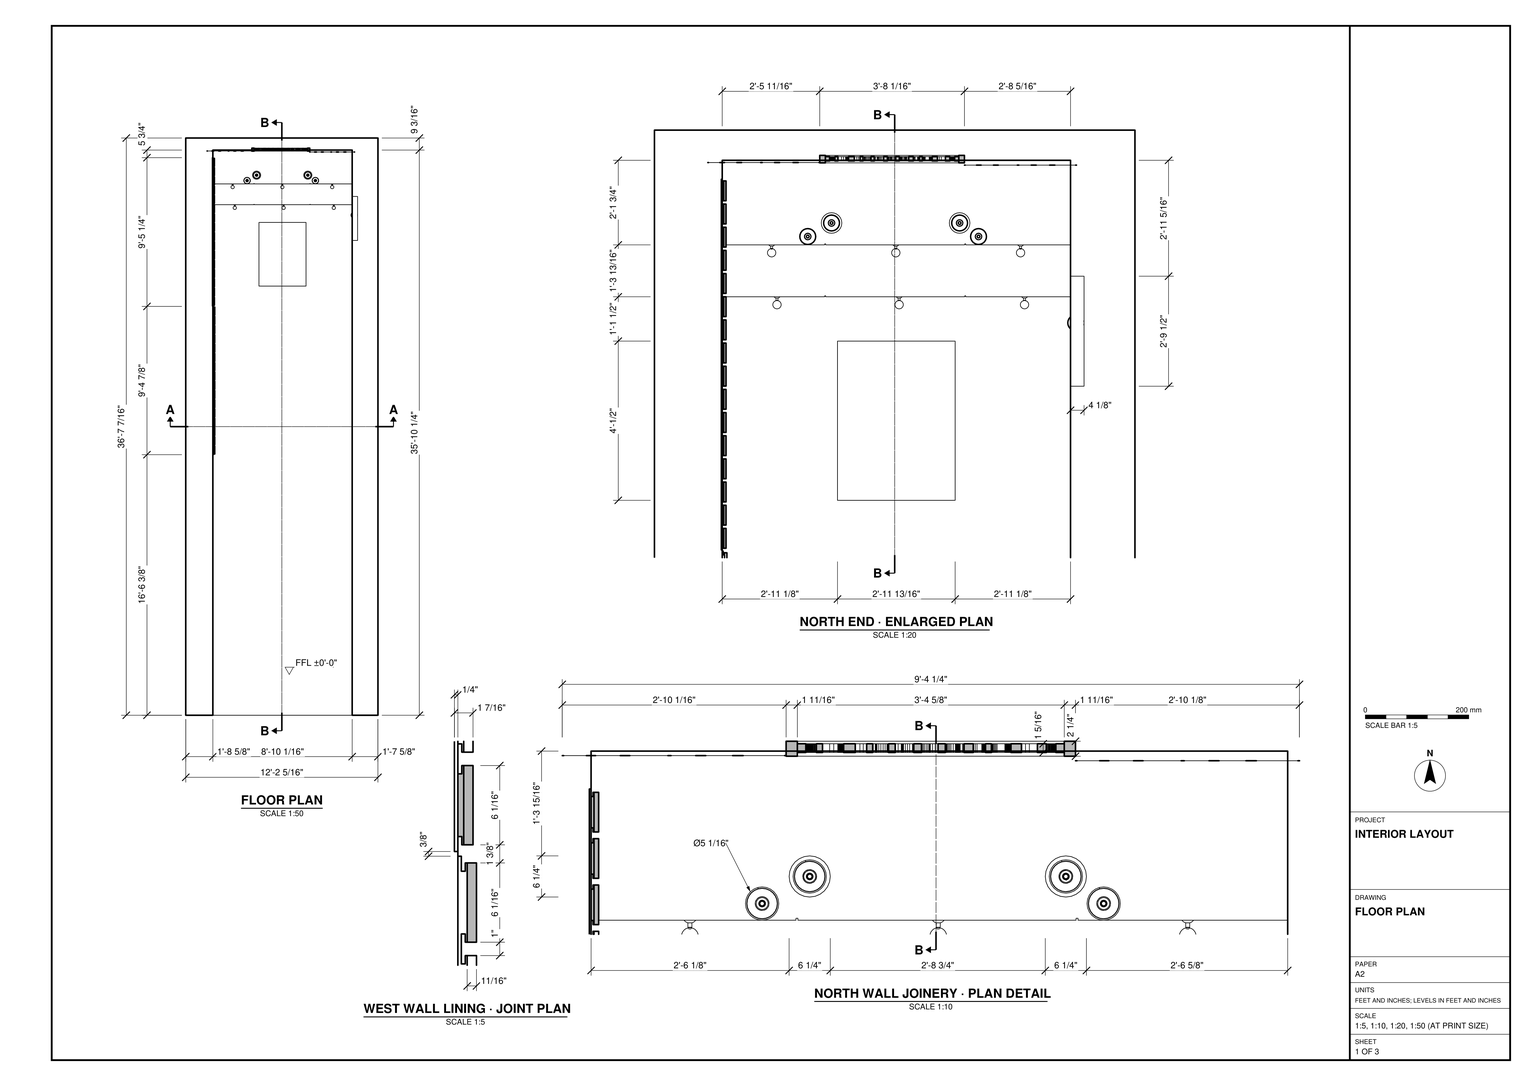
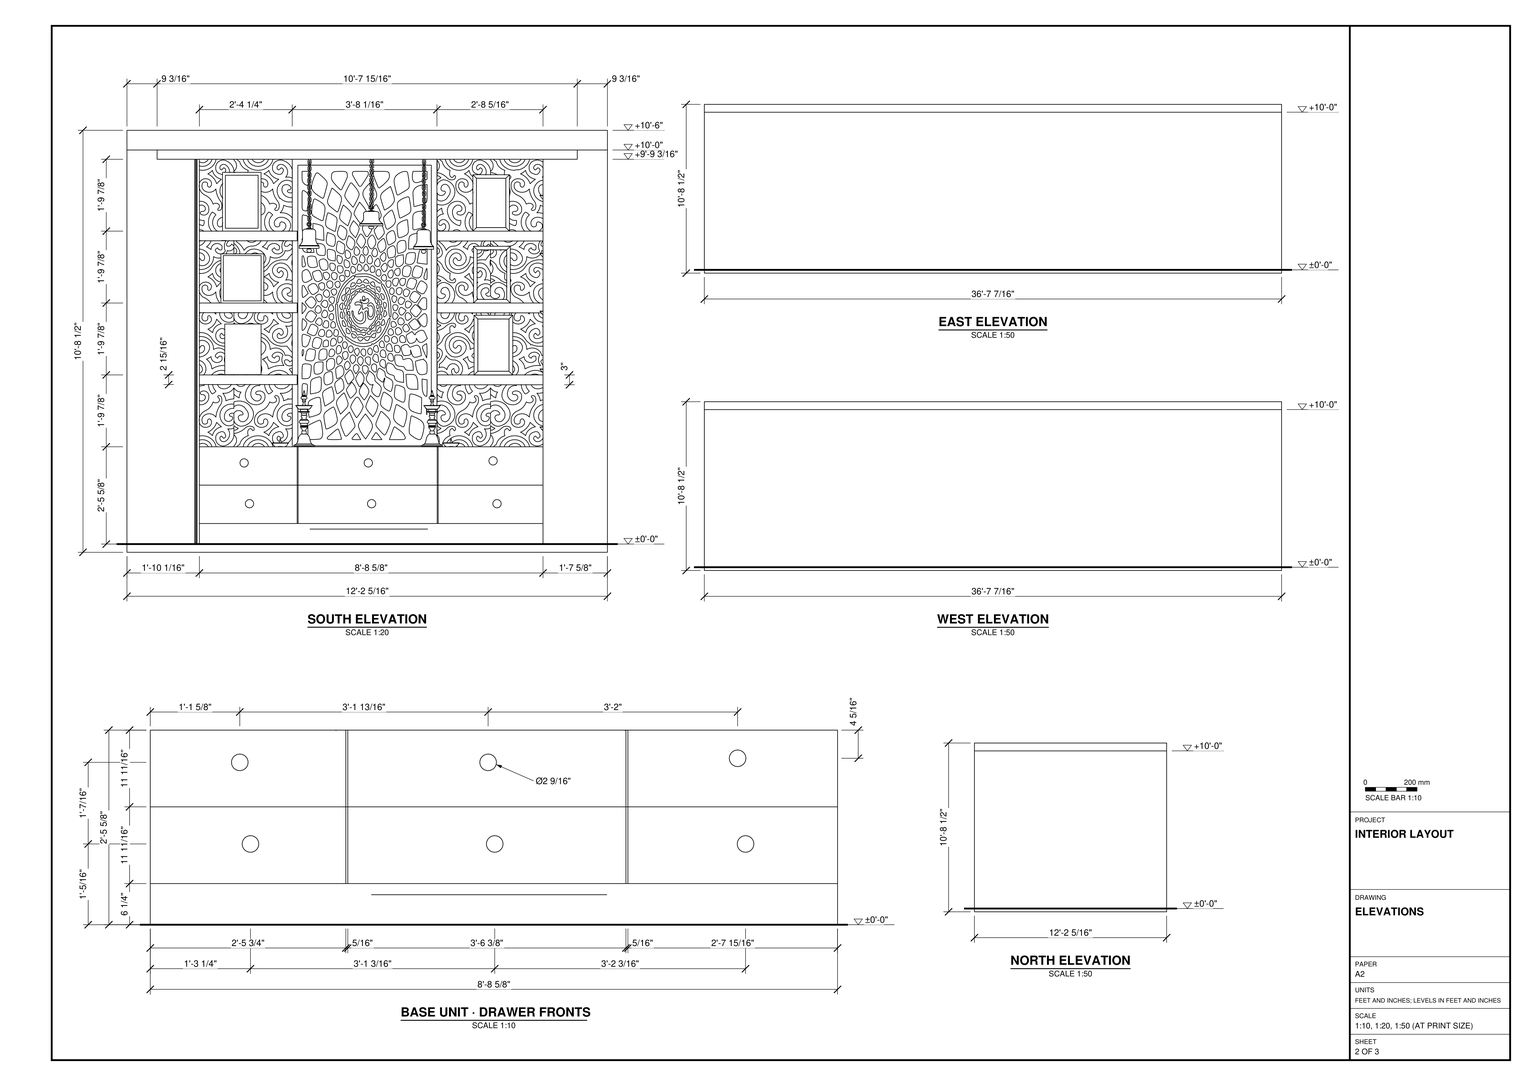
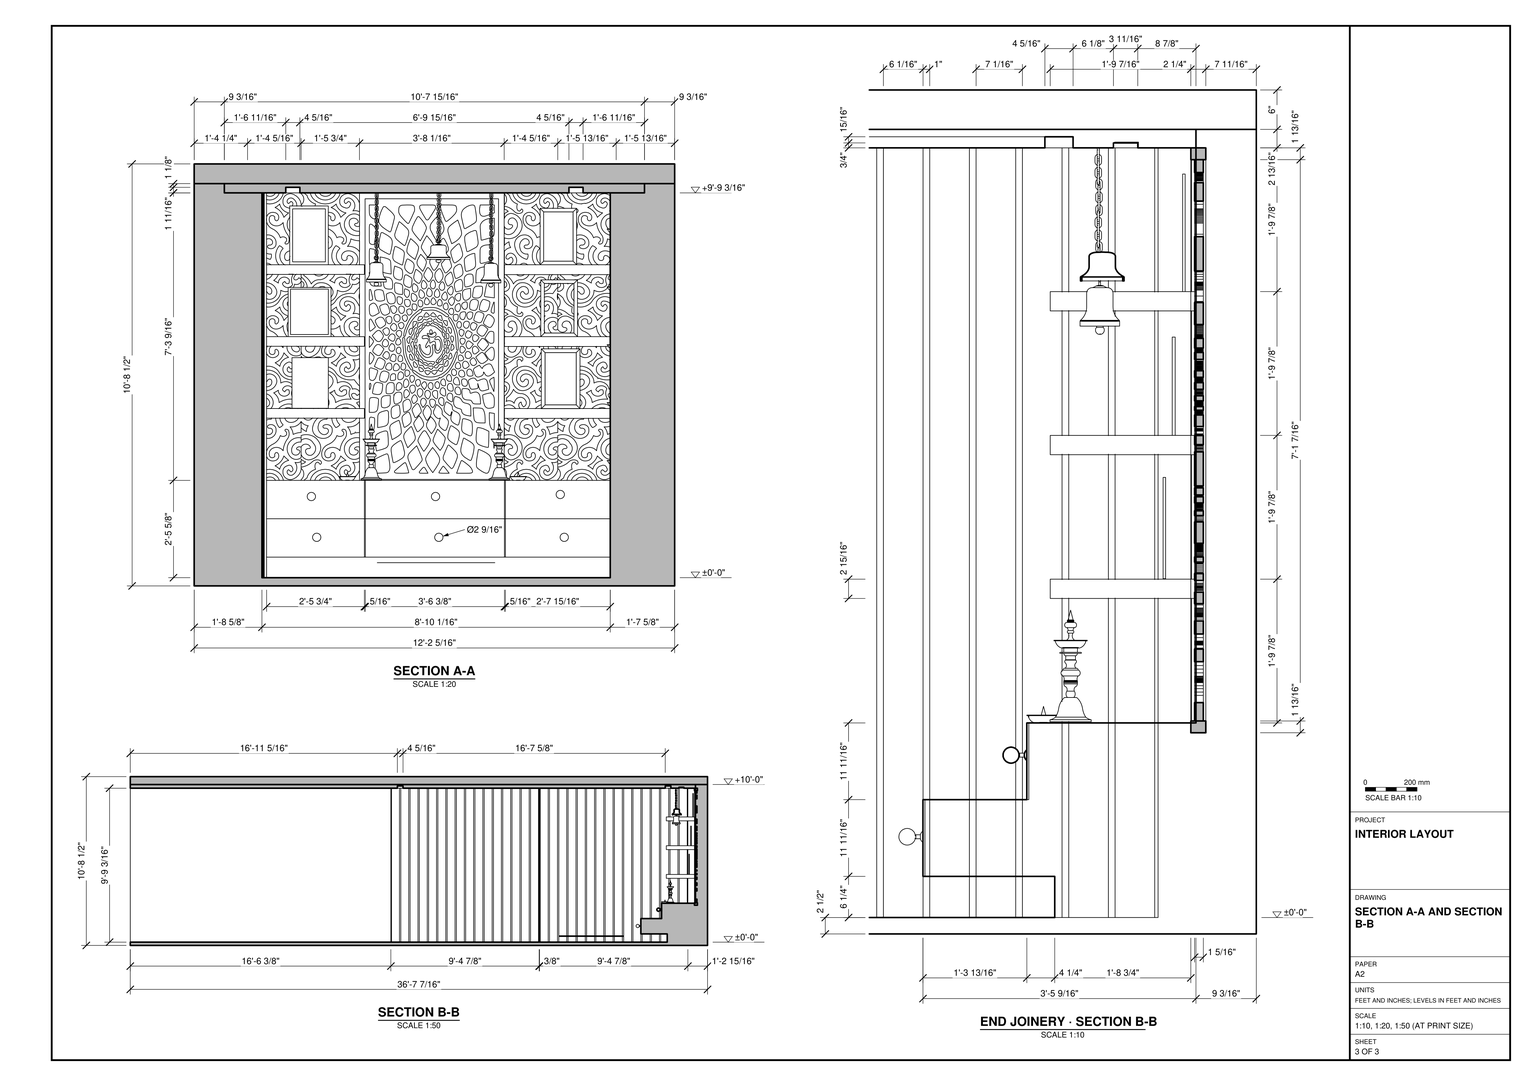
Build the interior in SketchUp from task_files/diagram_01.pdf. Work in feet and inches. Set the single finished floor level at ±0'-0". The overall model is 12'-2 5/16" wide from east to west, 36'-7 7/16" long from south to north and 10'-8 1/2" high.

Use the floor plan and sections to form the floor slab, side walls, north end wall and overhead slab at their drawn thicknesses. Keep the south end open. On the west wall, model the two runs of vertical lining toward the north end, following the joint detail; leave the approach from the south plain.

Build the north end base unit with a plinth, two rows of drawer fronts and round pulls. Use the enlarged longitudinal section for its stepped depth: the lower row projects farther into the room than the upper row. Above the base, place a tall patterned panel between two shelving bays. Give the middle panel its radial openwork and central medallion, and carry the scrolling pattern behind the side shelves. Place framed pictures on the shelves, lamps on the base, bells overhead and a rectangular rug on the floor in front of the display. Decor and loose items may be any suitable library components, for example from 3D Warehouse.

Keep the shell elements and each furniture or joinery piece in separate groups or components, and use components for repeated parts. Save one SketchUp model as output_files/prayer_room_with_built_in_display_joinery.skp.

# SketchUp Ruby script. Lengths in inches.
U = 1.inch
M = Sketchup.active_model
def pt(a) = Geom::Point3d.new(a.map { |v| v * U })
def face(e, loops, mat)
  f = e.add_face(loops[0].map { |a| pt(a) })
  loops[1..].each { |l| e.add_face(l.map { |a| pt(a) }).erase! }
  f.material = f.back_material = mat if mat
  f
end
# faces: each face lists its corners as indices into pts; further lists are holes
def faces(e, pts, list, mat = nil) = list.each { |f| face(e, (f[0].is_a?(Array) ? f : [f]).map { |l| l.map { |i| pts[i] } }, mat) }
# xy, xz, yz: faces in a plane at the given z, y or x. An outline is a flat list of corners, or four numbers for a rectangle; further outlines are holes
def ring(l) = l.size == 4 ? [[l[0], l[1]], [l[2], l[1]], [l[2], l[3]], [l[0], l[3]]] : l.each_slice(2).to_a
def flat(e, list, mat, &to3) = list.each { |f| face(e, (f[0].is_a?(Array) ? f : [f]).map { |l| ring(l).map { |u, v| to3.(u, v) } }, mat) }
def xy(e, z, list, mat = nil) = flat(e, list, mat) { |x, y| [x, y, z] }
def xz(e, y, list, mat = nil) = flat(e, list, mat) { |x, z| [x, y, z] }
def yz(e, x, list, mat = nil) = flat(e, list, mat) { |y, z| [x, y, z] }
def lines(e, pts, list) = list.each { |a, b| e.add_line(pt(pts[a]), pt(pts[b])) }
# prism: a flat outline (further loops are holes) pulled along v
def prism(e, loops, v, mat = nil)
  f = face(e, loops, mat); d = Geom::Vector3d.new(v.map { |x| x * U })
  f.pushpull(f.normal.samedirection?(d) ? d.length : -d.length)
end
def box(e, o, s, mat = nil) = prism(e, [[o, [o[0] + s[0], o[1], o[2]], [o[0] + s[0], o[1] + s[1], o[2]], [o[0], o[1] + s[1], o[2]]]], [0, 0, s[2]], mat)
def at(x, y, z, deg = 0) = Geom::Transformation.translation(pt([x, y, z])) * Geom::Transformation.rotation(ORIGIN, Z_AXIS, deg.degrees)
def axes(o, x, y, z) = Geom::Transformation.new([*x, 0, *y, 0, *z, 0, *pt(o).to_a, 1])
def part(name) = M.definitions.add(name)
# library, detail: a bought-in or finely detailed component or shape, given as its bounding box
def library(name, o, s) = part(name).tap { |d| box(d.entities, o, s) }
def detail(e, o, s) = box(e.add_group.entities, o, s)
def put(e, d, t, mat = nil) = e.add_instance(d, t).tap { |i| i.material = mat if mat }
def group(e, t, mat = nil) = e.add_group.tap { |g| g.transformation = t; g.material = mat if mat }.entities
root = M.entities
M.materials.add("[Color A01]1").color = [226, 181, 181]
M.materials.add("[Color B01]").color = [229, 193, 183]
M.materials.add("[Color C01]").color = [255, 229, 204]
M.materials.add("[Color C02]").color = [255, 204, 153]
M.materials.add("[Wood Veneer 02]").color = [190, 128, 91]
c1 = library("jali",[-1.5,-0.5,-1.5],[38.65,2,74.3])
c2 = library("Scrollwork panel",[0,0,0],[12.85,71.71,0.01])
c3 = library("bell",[83.36,153.84,-5.55],[7.09,7.09,33.42])
c4 = library("Deepam",[-1.66,-1.66,0],[3.32,3.32,9])
c5 = library("Globe wall light",[-0.72,0,-0.72],[5.39,5.72,5.38])
c6 = part("Framed panel")
xy(c6.entities,0,[[0,0,24.92,40.32]])
xy(c6.entities,1,[[[0,0,24.92,40.32],[1.38,1.74,23.35,38.95]],[1.38,1.74,23.35,38.95]])
xz(c6.entities,0,[[0,0,24.92,1]])
xz(c6.entities,40.32,[[0,0,24.92,1]])
yz(c6.entities,0,[[0,0,40.32,1]])
yz(c6.entities,24.92,[[0,0,40.32,1]])
c7 = part("GOD PHOTOFRAME")
box(c7.entities,[0,0,0],[24.57,34.27,0.85])
c8 = library("PHOTO FRAME",[-0.42,0,0],[1.15,22.25,34.37])
c9 = library("PHOTO FRAME\#1",[-0.42,0,0],[1.15,22.25,34.37])
c10 = library("PHOTO FRAME\#2",[-0.42,0,0],[1.15,22.25,34.37])
c11 = library("panel+ranurado",[0,-1.42,0],[48.03,1.42,96.0625])
c12 = part("Carpet+v15+(10)")
xy(c12.entities,0,[[0,0,118,159.69]])
c13 = library("Group\#21",[0,0,0],[5.07,5.07,2.53])
xy(root,0,[[0,0,146.3125,439.4375]])
xy(root,2.5,[[20.64,0,126.7,408.75]],"[Color A01]1")
xy(root,8.76,[[20.64,388.6875,20.64,408.75,126.7,408.75,126.7,388.6875,94.78,388.6875,94.78,388.99,94.48,388.99,94.48,388.6875,52.13,388.6875,52.13,388.99,51.83,388.99,51.83,388.6875]])
xy(root,20.45,[[20.64,388.6875,51.83,388.6875,51.83,388.99,52.13,388.99,52.13,388.6875,94.48,388.6875,94.48,388.99,94.78,388.99,94.78,388.6875,126.7,388.6875,126.7,404.5,94.78,404.5,94.78,404.8,94.48,404.8,94.48,404.5,52.13,404.5,52.13,404.8,51.83,404.8,51.83,404.5,20.64,404.5]],"[Color A01]1")
xy(root,32.13,[[20.64,404.5,51.83,404.5,51.83,404.8,52.13,404.8,52.13,404.5,94.48,404.5,94.48,404.8,94.78,404.8,94.78,404.5,126.7,404.5,126.7,430.25,20.64,430.25]],"[Color C01]")
xy(root,37,[[126.7,361.46,130.8125,394.96]],"[Color A01]1")
xy(root,49.1875,[[126.7,361.46,130.8125,394.96]])
xy(root,51.02,[[94.48,408.0625,126.7,430.25]],"[Color A01]1")
xy(root,51.08,[[20.64,408.0625,51.83,430.25]],"[Color A01]1")
xy(root,54.02,[[20.64,408.0625,51.83,430.25],[94.48,408.0625,126.7,430.25]],"[Color A01]1")
xy(root,54.625,[[126.7,361.46,130.8125,394.96]],"[Color A01]1")
xy(root,66.8125,[[126.7,361.46,130.8125,394.96]],"[Color A01]1")
xy(root,72.25,[[126.7,361.46,130.8125,394.96]])
xy(root,72.91,[[94.48,408.0625,126.7,430.25]],"[Color A01]1")
xy(root,72.97,[[20.64,408.0625,51.83,430.25]],"[Color A01]1")
xy(root,75.91,[[20.64,408.0625,51.83,430.25],[94.48,408.0625,126.7,430.25]])
xy(root,84.4375,[[126.7,361.46,130.8125,394.96]],"[Color A01]1")
xy(root,89.875,[[126.7,361.46,130.8125,394.96]])
xy(root,94.8,[[94.48,408.0625,126.7,430.25]],"[Color A01]1")
xy(root,94.86,[[20.64,408.0625,51.83,430.25]],"[Color A01]1")
xy(root,97.8,[[20.64,408.0625,51.83,430.25],[94.48,408.0625,126.7,430.25]])
xy(root,102.0625,[[126.7,361.46,130.8125,394.96]],"[Color A01]1")
xy(root,107.5,[[126.7,361.46,130.8125,394.96]])
xy(root,119.6875,[[9.1875,0,20.64,430.25],[126.7,0,126.7,361.46,130.8125,361.46,130.8125,394.96,126.7,394.96,126.7,430.25,137.125,430.25,137.125,0]])
xy(root,119.6875,[[[20.64,0,20.64,430.25,126.7,430.25,126.7,394.96,130.8125,394.96,130.8125,361.46,126.7,361.46,126.7,0],[27.9,203.33,118.42,411.54],[74.3,417.35,74.87,417.43,75.4,417.64,75.85,417.99,76.2,418.44,76.42,418.97,76.49,419.54,76.42,420.1,76.2,420.63,75.85,421.08,75.4,421.43,74.87,421.65,74.3,421.73,73.74,421.65,73.21,421.43,72.76,421.08,72.41,420.63,72.19,420.1,72.12,419.54,72.19,418.97,72.41,418.44,72.76,417.99,73.21,417.64,73.74,417.43],[118.85,417.87,119.32,417.92,119.76,418.08,120.15,418.35,120.45,418.72,120.65,419.15,120.73,419.62,120.68,420.09,120.52,420.53,120.24,420.92,119.88,421.22,119.45,421.42,118.98,421.5,118.51,421.45,118.07,421.29,117.68,421.01,117.38,420.65,117.18,420.22,117.1,419.75,117.15,419.28,117.3125,418.84,117.59,418.45,117.95,418.15,118.38,417.95],[27.1,417.87,27.57,417.92,28.01,418.08,28.4,418.35,28.7,418.72,28.9,419.15,28.98,419.62,28.93,420.09,28.77,420.53,28.49,420.92,28.13,421.22,27.7,421.42,27.23,421.5,26.76,421.45,26.32,421.29,25.93,421.01,25.63,420.65,25.43,420.22,25.35,419.75,25.4,419.28,25.5625,418.84,25.84,418.45,26.2,418.15,26.63,417.95]],[32.1875,207.625,114.125,407.25]],"[Color A01]1")
xy(root,120.4375,[[74.3,417.35,73.74,417.43,73.21,417.64,72.76,417.99,72.41,418.44,72.19,418.97,72.12,419.54,72.19,420.1,72.41,420.63,72.76,421.08,73.21,421.43,73.74,421.65,74.3,421.73,74.87,421.65,75.4,421.43,75.85,421.08,76.2,420.63,76.42,420.1,76.49,419.54,76.42,418.97,76.2,418.44,75.85,417.99,75.4,417.64,74.87,417.43]])
xy(root,120.5625,[[27.1,417.87,26.63,417.95,26.2,418.15,25.84,418.45,25.5625,418.84,25.4,419.28,25.35,419.75,25.43,420.22,25.63,420.65,25.93,421.01,26.32,421.29,26.76,421.45,27.23,421.5,27.7,421.42,28.13,421.22,28.49,420.92,28.77,420.53,28.93,420.09,28.98,419.62,28.9,419.15,28.7,418.72,28.4,418.35,28.01,418.08,27.57,417.92],[118.85,417.87,118.38,417.95,117.95,418.15,117.59,418.45,117.3125,418.84,117.15,419.28,117.1,419.75,117.18,420.22,117.38,420.65,117.68,421.01,118.07,421.29,118.51,421.45,118.98,421.5,119.45,421.42,119.88,421.22,120.24,420.92,120.52,420.53,120.68,420.09,120.73,419.62,120.65,419.15,120.45,418.72,120.15,418.35,119.76,418.08,119.32,417.92]])
xy(root,121.375,[[[27.9,203.33,118.42,411.54],[32.1875,207.625,114.125,407.25]]],"[Color A01]1")
xy(root,122.5,[[0,0,0,439.4375,146.3125,439.4375,146.3125,0,137.125,0,137.125,430.25,9.1875,430.25,9.1875,0],[9.1875,0,137.125,430.25]])
xy(root,128.5,[[0,0,146.3125,439.4375]])
xz(root,0,[[0,0,146.3125,0,146.3125,122.5,137.125,122.5,137.125,119.6875,126.7,119.6875,126.7,2.5,20.64,2.5,20.64,119.6875,9.1875,119.6875,9.1875,122.5,0,122.5],[9.1875,119.6875,137.125,122.5],[0,122.5,146.3125,128.5]])
xz(root,203.33,[[27.9,119.6875,118.42,121.375]])
xz(root,207.625,[[32.1875,119.6875,114.125,121.375]])
xz(root,361.46,[[126.7,37,130.8125,49.1875],[126.7,54.625,130.8125,66.8125],[126.7,72.25,130.8125,84.4375],[126.7,89.875,130.8125,102.0625],[126.7,107.5,130.8125,119.6875]])
xz(root,388.6875,[[20.64,8.76,51.83,20.45],[52.13,8.76,94.48,20.45],[94.78,8.76,126.7,20.45]],"[Color A01]1")
xz(root,388.99,[[51.83,8.76,52.13,20.45],[94.48,8.76,94.78,20.45]])
xz(root,394.96,[[126.7,37,130.8125,49.1875],[126.7,54.625,130.8125,66.8125],[126.7,72.25,130.8125,84.4375],[126.7,89.875,130.8125,102.0625],[126.7,107.5,130.8125,119.6875]],"[Color A01]1")
xz(root,404.5,[[20.64,20.45,51.83,32.13],[52.13,20.45,94.48,32.13],[94.78,20.45,126.7,32.13]],"[Color A01]1")
xz(root,404.8,[[51.83,20.45,52.13,32.13],[94.48,20.45,94.78,32.13]])
xz(root,407.25,[[32.1875,119.6875,114.125,121.375]])
xz(root,408.0625,[[94.48,51.02,126.7,54.02],[20.64,51.08,51.83,54.02],[94.48,72.91,126.7,75.91],[20.64,72.97,51.83,75.91],[94.48,94.8,126.7,97.8],
  [20.64,94.86,51.83,97.8]],"[Color A01]1")
xz(root,408.75,[[20.64,2.5,126.7,8.76]],"[Color A01]1")
xz(root,411.54,[[27.9,119.6875,118.42,121.375]],"[Color A01]1")
xz(root,430.25,[[9.1875,119.6875,137.125,122.5]])
xz(root,430.25,[[20.64,32.13,51.83,51.08],[51.83,32.13,94.48,119.6875],[94.48,32.13,126.7,51.02],[20.64,54.02,51.83,72.97],[94.48,54.02,126.7,72.91],
  [20.64,75.91,51.83,94.86],[94.48,75.91,126.7,94.8],[20.64,97.8,51.83,119.6875],[94.48,97.8,126.7,119.6875]],"[Color B01]")
xz(root,439.4375,[[0,0,146.3125,122.5],[0,122.5,146.3125,128.5]])
yz(root,0,[[0,0,439.4375,122.5],[0,122.5,439.4375,128.5]])
yz(root,9.1875,[[0,119.6875,430.25,122.5]])
yz(root,20.64,[[0,2.5,408.75,2.5,408.75,8.76,388.6875,8.76,388.6875,20.45,404.5,20.45,404.5,32.13,430.25,32.13,430.25,51.08,408.0625,51.08,408.0625,54.02,430.25,54.02,430.25,72.97,408.0625,72.97,408.0625,75.91,430.25,75.91,430.25,94.86,408.0625,94.86,408.0625,97.8,430.25,97.8,430.25,119.6875,0,119.6875]],"[Color A01]1")
yz(root,27.9,[[203.33,119.6875,411.54,121.375]],"[Color A01]1")
yz(root,32.1875,[[207.625,119.6875,407.25,121.375]])
yz(root,51.83,[[388.6875,8.76,388.99,20.45],[404.5,20.45,404.8,32.13],[408.0625,51.08,430.25,54.02],[408.0625,72.97,430.25,75.91]])
yz(root,51.83,[[408.0625,94.86,430.25,97.8]],"[Color A01]1")
yz(root,52.13,[[388.6875,8.76,388.99,20.45],[404.5,20.45,404.8,32.13]])
yz(root,94.48,[[388.6875,8.76,388.99,20.45],[404.5,20.45,404.8,32.13],[408.0625,51.02,430.25,54.02],[408.0625,72.91,430.25,75.91],[408.0625,94.8,430.25,97.8]])
yz(root,94.78,[[388.6875,8.76,388.99,20.45],[404.5,20.45,404.8,32.13]])
yz(root,114.125,[[207.625,119.6875,407.25,121.375]])
yz(root,118.42,[[203.33,119.6875,411.54,121.375]],"[Color A01]1")
yz(root,126.7,[[[0,2.5,0,119.6875,361.46,119.6875,361.46,107.5,394.96,107.5,394.96,119.6875,430.25,119.6875,430.25,97.8,408.0625,97.8,408.0625,94.8,430.25,94.8,430.25,75.91,408.0625,75.91,408.0625,72.91,430.25,72.91,430.25,54.02,408.0625,54.02,408.0625,51.02,430.25,51.02,430.25,32.13,404.5,32.13,404.5,20.45,388.6875,20.45,388.6875,8.76,408.75,8.76,408.75,2.5],[361.46,89.875,394.96,102.0625],[361.46,72.25,394.96,84.4375],[361.46,54.625,394.96,66.8125],[361.46,37,394.96,49.1875]]],"[Color A01]1")
yz(root,130.8125,[[361.46,37,394.96,49.1875],[361.46,54.625,394.96,66.8125],[361.46,72.25,394.96,84.4375],[361.46,89.875,394.96,102.0625],[361.46,107.5,394.96,119.6875]],"[Color A01]1")
yz(root,137.125,[[0,119.6875,430.25,122.5]])
yz(root,146.3125,[[0,0,439.4375,122.5],[0,122.5,439.4375,128.5]])
p = [[73.74,417.43,119.6875],[73.21,417.64,119.6875],[73.21,417.64,120.4375],[73.74,417.43,120.4375],[74.3,417.35,119.6875],[74.3,417.35,120.4375],
  [74.87,417.43,119.6875],[74.87,417.43,120.4375],[75.4,417.64,119.6875],[75.4,417.64,120.4375],[72.76,417.99,119.6875],[72.76,417.99,120.4375],
  [75.85,417.99,119.6875],[75.85,417.99,120.4375],[27.1,417.87,119.6875],[26.63,417.95,119.6875],[26.63,417.95,120.5625],[27.1,417.87,120.5625],
  [27.57,417.92,119.6875],[27.57,417.92,120.5625],[28.01,418.08,119.6875],[28.01,418.08,120.5625],[118.85,417.87,119.6875],[118.38,417.95,119.6875],
  [118.38,417.95,120.5625],[118.85,417.87,120.5625],[119.32,417.92,119.6875],[119.32,417.92,120.5625],[119.76,418.08,119.6875],[119.76,418.08,120.5625],
  [26.2,418.15,119.6875],[26.2,418.15,120.5625],[72.41,418.44,119.6875],[72.41,418.44,120.4375],[76.2,418.44,119.6875],[76.2,418.44,120.4375],
  [117.95,418.15,119.6875],[117.95,418.15,120.5625],[25.84,418.45,119.6875],[25.84,418.45,120.5625],[28.4,418.35,119.6875],[28.4,418.35,120.5625],
  [117.59,418.45,119.6875],[117.59,418.45,120.5625],[120.15,418.35,119.6875],[120.15,418.35,120.5625],[28.7,418.72,119.6875],[28.7,418.72,120.5625],
  [72.19,418.97,119.6875],[72.19,418.97,120.4375],[76.42,418.97,119.6875],[76.42,418.97,120.4375],[120.45,418.72,119.6875],[120.45,418.72,120.5625],
  [25.5625,418.84,119.6875],[25.5625,418.84,120.5625],[117.3125,418.84,119.6875],[117.3125,418.84,120.5625],[28.9,419.15,119.6875],[28.9,419.15,120.5625],
  [120.65,419.15,119.6875],[120.65,419.15,120.5625],[25.4,419.28,119.6875],[25.4,419.28,120.5625],[117.15,419.28,119.6875],[117.15,419.28,120.5625],
  [72.12,419.54,119.6875],[72.12,419.54,120.4375],[76.49,419.54,119.6875],[76.49,419.54,120.4375],[28.98,419.62,119.6875],[28.98,419.62,120.5625],
  [120.73,419.62,119.6875],[120.73,419.62,120.5625],[25.35,419.75,119.6875],[25.35,419.75,120.5625],[117.1,419.75,119.6875],[117.1,419.75,120.5625],
  [72.19,420.1,119.6875],[72.19,420.1,120.4375],[76.42,420.1,119.6875],[76.42,420.1,120.4375],[28.93,420.09,119.6875],[28.93,420.09,120.5625],
  [120.68,420.09,119.6875],[120.68,420.09,120.5625],[25.43,420.22,119.6875],[25.43,420.22,120.5625],[117.18,420.22,119.6875],[117.18,420.22,120.5625],
  [28.77,420.53,119.6875],[28.77,420.53,120.5625],[72.41,420.63,119.6875],[72.41,420.63,120.4375],[76.2,420.63,119.6875],[76.2,420.63,120.4375],
  [120.52,420.53,119.6875],[120.52,420.53,120.5625],[25.63,420.65,119.6875],[25.63,420.65,120.5625],[117.38,420.65,119.6875],[117.38,420.65,120.5625],
  [28.49,420.92,119.6875],[28.49,420.92,120.5625],[120.24,420.92,119.6875],[120.24,420.92,120.5625],[25.93,421.01,119.6875],[25.93,421.01,120.5625],
  [72.76,421.08,119.6875],[72.76,421.08,120.4375],[75.85,421.08,119.6875],[75.85,421.08,120.4375],[117.68,421.01,119.6875],[117.68,421.01,120.5625],
  [28.13,421.22,119.6875],[28.13,421.22,120.5625],[119.88,421.22,119.6875],[119.88,421.22,120.5625],[26.32,421.29,119.6875],[26.32,421.29,120.5625],
  [118.07,421.29,119.6875],[118.07,421.29,120.5625],[73.21,421.43,119.6875],[73.21,421.43,120.4375],[75.4,421.43,119.6875],[75.4,421.43,120.4375],
  [27.7,421.42,119.6875],[27.7,421.42,120.5625],[119.45,421.42,119.6875],[119.45,421.42,120.5625],[26.76,421.45,119.6875],[26.76,421.45,120.5625],
  [118.51,421.45,119.6875],[118.51,421.45,120.5625],[27.23,421.5,119.6875],[27.23,421.5,120.5625],[73.74,421.65,119.6875],[73.74,421.65,120.4375],
  [74.87,421.65,119.6875],[74.87,421.65,120.4375],[118.98,421.5,119.6875],[118.98,421.5,120.5625],[74.3,421.73,119.6875],[74.3,421.73,120.4375]]
faces(root,p,[[0,1,2,3],[4,0,3,5],[6,4,5,7],[8,6,7,9],[1,10,11,2],[12,8,9,13],[14,15,16,17],[18,14,17,19],
  [20,18,19,21],[22,23,24,25],[26,22,25,27],[28,26,27,29],[15,30,31,16],[10,32,33,11],[34,12,13,35],[23,36,37,24],
  [30,38,39,31],[40,20,21,41],[36,42,43,37],[44,28,29,45],[46,40,41,47],[32,48,49,33],[50,34,35,51],[52,44,45,53],
  [38,54,55,39],[42,56,57,43],[58,46,47,59],[60,52,53,61],[54,62,63,55],[56,64,65,57],[48,66,67,49],[68,50,51,69],
  [70,58,59,71],[72,60,61,73],[62,74,75,63],[64,76,77,65],[66,78,79,67],[80,68,69,81],[82,70,71,83],[84,72,73,85],
  [74,86,87,75],[76,88,89,77],[90,82,83,91],[78,92,93,79],[94,80,81,95],[96,84,85,97],[86,98,99,87],[88,100,101,89],
  [102,90,91,103],[104,96,97,105],[98,106,107,99],[92,108,109,93],[110,94,95,111],[100,112,113,101],[114,102,103,115],[116,104,105,117],
  [106,118,119,107],[112,120,121,113],[108,122,123,109],[124,110,111,125],[126,114,115,127],[128,116,117,129],[118,130,131,119],[120,132,133,121],
  [134,126,127,135],[122,136,137,123],[138,124,125,139],[140,128,129,141],[130,134,135,131],[132,140,141,133],[136,142,143,137],[142,138,139,143]])
put(root,c1,axes([52.04,430.04,32.43],[1.14,0,0],[0,1.14,0],[0,0,1.19868]))
put(root,c2,axes([16.25,429.5625,32.13],[1.27,0,0],[0,0,1.22097],[0,-1,0]))
put(root,c2,axes([32.57,429.5625,32.13],[1.38453,0,0],[0,0,1.22097],[0,-1,0]),"[Color B01]")
put(root,c2,axes([110.71,428.78,32.13],[1.38453,0,0],[0,0,1.22097],[0,-1,0]),"[Color C02]")
put(root,c2,axes([94.39,428.78,32.13],[1.27,0,0],[0,0,1.22097],[0,-1,0]))
put(root,c3,axes([-18.4,281.84,95.99],[0.85,0,0],[0,0.85,0],[0,0,0.85]))
put(root,c3,axes([-12.5,258.6,102],[1,0,0],[0,1,0],[0,0,0.63455]))
put(root,c3,axes([15.74,281.37,95.76],[0.8585,0,0],[0,0.8585,0],[0,0,0.8585]))
put(root,c4,axes([53.92,411.16,32.3],[1.89,0,0],[0,1.89,0],[0,0,1.89]))
put(root,c5,axes([36.95,400.83,28.49],[-0.6426,0,0],[0,0.6426,0],[0,0,-0.6426]))
put(root,c5,axes([74.77,400.83,28.49],[-0.6426,0,0],[0,0.6426,0],[0,0,-0.6426]))
put(root,c5,axes([112.75,400.83,29.11],[-0.6426,0,0],[0,0.6426,0],[0,0,-0.6426]))
put(root,c5,axes([38.58,385.02,16.0625],[-0.6426,0,0],[0,0.6426,0],[0,0,-0.6426]))
put(root,c5,axes([75.77,385.02,16.0625],[-0.6426,0,0],[0,0.6426,0],[0,0,-0.6426]))
put(root,c5,axes([113.96,385.02,16.0625],[-0.6426,0,0],[0,0.6426,0],[0,0,-0.6426]))
put(root,c6,axes([28.62,427.09,75.91],[0.5244,0,0],[0,0,0.37131],[0,-0.44844,0]))
put(root,c7,axes([29.79,425.63,54.09],[0.45,0,0],[0,0,0.45],[0,-0.45,0]))
put(root,c8,axes([105.55,428.09,75.91],[0,0.60348,0],[0.5029,0,0],[0,0,0.5029]))
put(root,c9,axes([105.34,422.59,97.8],[0,0.06,0],[0.5,0,0],[0,0,0.5]))
put(root,c10,axes([105.7,425.79,53.98],[0,1.1978,0],[0.53,0,0],[0,0,0.53]))
put(root,c11,axes([20.375,311.61,2.5],[0,2.35,0],[-1,0,0],[0,0,1.2199]))
put(root,c11,axes([20.64,198.375,2.5],[0,2.35,0],[-1,0,0],[0,0,1.2199]))
put(root,c4,axes([92.92,411.16,32.3],[1.89,0,0],[0,1.89,0],[0,0,1.89]))
put(root,c12,axes([55.74,326.7,7.07],[0.3036,0,0],[0,0.3036,0],[0,0,0.3036]))
put(root,c13,at(44.14,404.5,32.13))
put(root,c13,at(96.14,404.5,32.13))
put(root,c13,at(125.74,378.21,72.25))
put(root,c13,at(125.74,378.21,54.625))
put(root,c13,at(125.74,378.21,37))
put(root,c13,at(125.74,378.21,89.875))
put(root,c13,at(125.74,378.21,107.5))
g1 = group(root,at(29.09,428.6,115.7),"[Wood Veneer 02]")
xy(g1,-17.91,[[0,-0.38,11.74,0]])
xy(g1,-17.02,[[0.89,-0.38,10.86,0]])
xy(g1,-0.89,[[0.89,-0.38,10.86,0]])
xy(g1,0,[[0,-0.38,11.74,0]])
xz(g1,-0.38,[[[0,-17.91,11.74,0],[0.89,-17.02,10.86,-0.89]]])
xz(g1,0,[[[0,-17.91,11.74,0],[0.89,-17.02,10.86,-0.89]],[0.89,-17.02,10.86,-0.89]])
yz(g1,0,[[-0.38,-17.91,0,0]])
yz(g1,0.89,[[-0.38,-17.02,0,-0.89]])
yz(g1,10.86,[[-0.38,-17.02,0,-0.89]])
yz(g1,11.74,[[-0.38,-17.91,0,0]])
